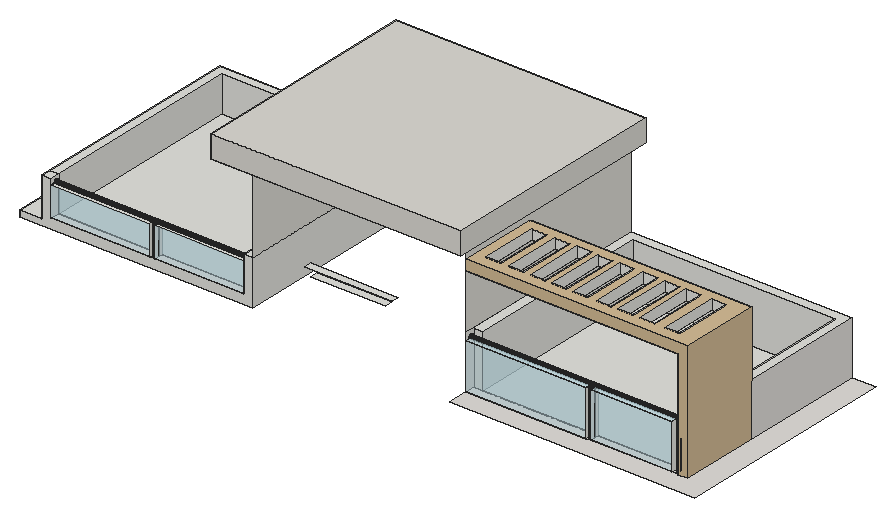
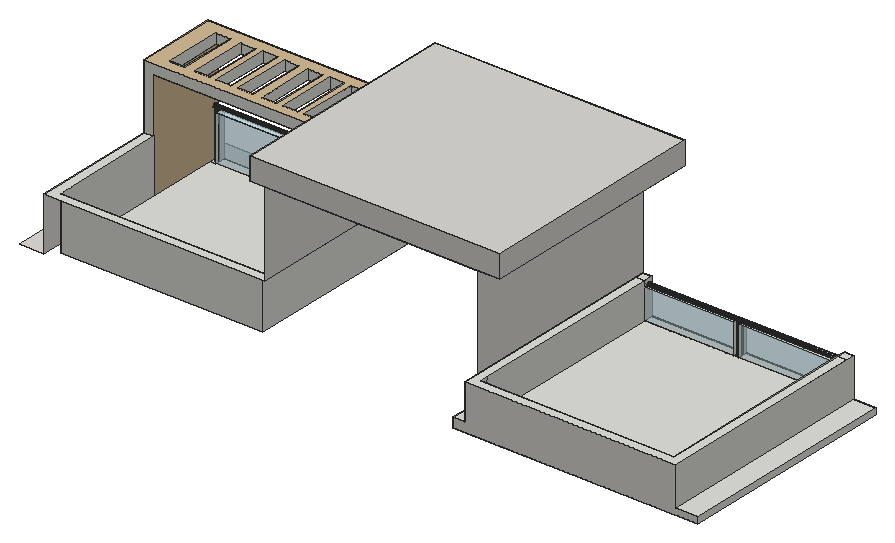
# SketchUp Ruby script. Lengths in inches.
U = 1.inch
M = Sketchup.active_model
def pt(a) = Geom::Point3d.new(a.map { |v| v * U })
def face(e, loops, mat)
  f = e.add_face(loops[0].map { |a| pt(a) })
  loops[1..].each { |l| e.add_face(l.map { |a| pt(a) }).erase! }
  f.material = f.back_material = mat if mat
  f
end
# faces: each face lists its corners as indices into pts; further lists are holes
def faces(e, pts, list, mat = nil) = list.each { |f| face(e, (f[0].is_a?(Array) ? f : [f]).map { |l| l.map { |i| pts[i] } }, mat) }
# xy, xz, yz: faces in a plane at the given z, y or x. An outline is a flat list of corners, or four numbers for a rectangle; further outlines are holes
def ring(l) = l.size == 4 ? [[l[0], l[1]], [l[2], l[1]], [l[2], l[3]], [l[0], l[3]]] : l.each_slice(2).to_a
def flat(e, list, mat, &to3) = list.each { |f| face(e, (f[0].is_a?(Array) ? f : [f]).map { |l| ring(l).map { |u, v| to3.(u, v) } }, mat) }
def xy(e, z, list, mat = nil) = flat(e, list, mat) { |x, y| [x, y, z] }
def xz(e, y, list, mat = nil) = flat(e, list, mat) { |x, z| [x, y, z] }
def yz(e, x, list, mat = nil) = flat(e, list, mat) { |y, z| [x, y, z] }
def lines(e, pts, list) = list.each { |a, b| e.add_line(pt(pts[a]), pt(pts[b])) }
# prism: a flat outline (further loops are holes) pulled along v
def prism(e, loops, v, mat = nil)
  f = face(e, loops, mat); d = Geom::Vector3d.new(v.map { |x| x * U })
  f.pushpull(f.normal.samedirection?(d) ? d.length : -d.length)
end
def box(e, o, s, mat = nil) = prism(e, [[o, [o[0] + s[0], o[1], o[2]], [o[0] + s[0], o[1] + s[1], o[2]], [o[0], o[1] + s[1], o[2]]]], [0, 0, s[2]], mat)
def at(x, y, z, deg = 0) = Geom::Transformation.translation(pt([x, y, z])) * Geom::Transformation.rotation(ORIGIN, Z_AXIS, deg.degrees)
def axes(o, x, y, z) = Geom::Transformation.new([*x, 0, *y, 0, *z, 0, *pt(o).to_a, 1])
def part(name) = M.definitions.add(name)
# library, detail: a bought-in or finely detailed component or shape, given as its bounding box
def library(name, o, s) = part(name).tap { |d| box(d.entities, o, s) }
def detail(e, o, s) = box(e.add_group.entities, o, s)
def put(e, d, t, mat = nil) = e.add_instance(d, t).tap { |i| i.material = mat if mat }
def group(e, t, mat = nil) = e.add_group.tap { |g| g.transformation = t; g.material = mat if mat }.entities
root = M.entities
M.materials.add("[Formica Beige]").color = [211, 187, 149]
M.materials.add("[Terrazzo Tile Accent]").color = [224, 221, 217]
M.materials.add("[Terrazzo Tile Light]").color = [219, 217, 210]
M.materials.add("[Translucent Glass Safety]").color = [204, 235, 244]
M.materials["[Translucent Glass Safety]"].alpha = 0.5
xy(root,573.6875,[[8.45,114.1,21.57,244.83],[21.57,114.1,21.57,244.83,152.39,244.83,152.39,235.11,145.58,235.11,145.58,114.1],[270.97,114.1,270.97,119.66,341.44,119.66,341.44,117.58,341.3125,117.27,341.27,116.91,341.3125,116.56,341.44,116.24,341.44,114.1],[341.44,114.1,344.2,114.1,344.2,119.66,341.44,119.66,341.44,117.58,341.45,117.6,341.67,117.88,341.95,118.1,342.29,118.24,342.64,118.29,343,118.24,343.33,118.1,343.61,117.88,343.83,117.6,343.97,117.27,344.02,116.91,343.97,116.56,343.83,116.22,343.61,115.9375,343.33,115.72,343,115.58,342.64,115.54,342.29,115.58,341.95,115.72,341.67,115.9375,341.45,116.22,341.44,116.24],[344.2,114.1,391.99,119.66],
  [[391.99,114.1,395.61,119.66],[393.42,116.1875,393.17,116.22,392.92,116.32,392.72,116.48,392.56,116.6875,392.46,116.93,392.42,117.1875,392.46,117.45,392.56,117.6875,392.72,117.89,392.92,118.05,393.17,118.15,393.42,118.1875,393.68,118.15,393.92,118.05,394.13,117.89,394.29,117.6875,394.39,117.45,394.42,117.1875,394.39,116.93,394.29,116.6875,394.13,116.48,393.92,116.32,393.68,116.22]],[342.64,115.54,342.29,115.58,341.95,115.72,341.67,115.9375,341.45,116.22,341.44,116.24,341.44,117.58,341.45,117.6,341.67,117.88,341.95,118.1,342.29,118.24,342.64,118.29,343,118.24,343.33,118.1,343.61,117.88,343.83,117.6,343.97,117.27,344.02,116.91,343.97,116.56,343.83,116.22,343.61,115.9375,343.33,115.72,343,115.58],[393.42,116.1875,393.17,116.22,392.92,116.32,392.72,116.48,392.56,116.6875,392.46,116.93,392.42,117.1875,392.46,117.45,392.56,117.6875,392.72,117.89,392.92,118.05,393.17,118.15,393.42,118.1875,393.68,118.15,393.92,118.05,394.13,117.89,394.29,117.6875,394.39,117.45,394.42,117.1875,394.39,116.93,394.29,116.6875,394.13,116.48,393.92,116.32,393.68,116.22],[341.44,116.24,341.3125,116.56,341.27,116.91,341.3125,117.27,341.44,117.58],[276.53,119.66,395.61,229.56]])
xy(root,573.6875,[[270.97,102.04,415.04,102.04,415.04,235.11,401.16,235.11,401.16,114.1,270.97,114.1]],"[Terrazzo Tile Accent]")
xy(root,577.14,[[8.45,114.1,21.57,244.83]])
xy(root,579.1875,[[26.86,114.1,84.93,119.4],[[84.93,114.1,87.68,119.4],[86.24,115.7,85.92,115.74,85.62,115.86,85.36,116.0625,85.16,116.32,85.04,116.625,84.99,116.95,85.04,117.27,85.16,117.57,85.36,117.83,85.62,118.03,85.92,118.15,86.24,118.2,86.57,118.15,86.87,118.03,87.13,117.83,87.33,117.57,87.45,117.27,87.49,116.95,87.45,116.625,87.33,116.32,87.13,116.0625,86.87,115.86,86.57,115.74]],[87.68,114.1,140.28,119.4],[86.24,115.7,85.92,115.74,85.62,115.86,85.36,116.0625,85.16,116.32,85.04,116.625,84.99,116.95,85.04,117.27,85.16,117.57,85.36,117.83,85.62,118.03,85.92,118.15,86.24,118.2,86.57,118.15,86.87,118.03,87.13,117.83,87.33,117.57,87.45,117.27,87.49,116.95,87.45,116.625,87.33,116.32,87.13,116.0625,86.87,115.86,86.57,115.74],[26.86,119.4,140.28,239.54]])
xy(root,579.1875,[[145.58,235.11,152.39,244.83]],"[Terrazzo Tile Accent]")
xy(root,596.84,[[26.86,114.1,84.93,116.21],[87.68,114.1,140.28,116.21],[26.86,116.21,84.93,117.71],[87.68,116.21,140.28,117.71],[26.86,117.71,84.93,119.4],
  [87.68,117.71,140.28,119.4]])
xy(root,597.4375,[[86.24,115.7,86.57,115.74,86.87,115.86,87.13,116.0625,87.33,116.32,87.45,116.625,87.49,116.95,87.45,117.27,87.33,117.57,87.13,117.83,86.87,118.03,86.57,118.15,86.24,118.2,85.92,118.15,85.62,118.03,85.36,117.83,85.16,117.57,85.04,117.27,84.99,116.95,85.04,116.625,85.16,116.32,85.36,116.0625,85.62,115.86,85.92,115.74]])
xy(root,600.1875,[[21.57,114.1,26.86,119.4],[140.28,114.1,145.58,119.4],[21.57,119.4,26.86,119.4,26.86,239.54,140.28,239.54,140.28,119.4,145.58,119.4,145.58,244.83,21.57,244.83]])
xy(root,600.1875,[[270.97,114.1,341.44,114.1,341.44,116.24,341.3125,116.56,341.27,116.91,341.3125,117.27,341.44,117.58,341.44,119.66,270.97,119.66],[344.2,114.1,391.99,119.66]],"[Translucent Glass Safety]")
xy(root,601.4375,[[393.42,116.1875,393.68,116.22,393.92,116.32,394.13,116.48,394.29,116.6875,394.39,116.93,394.42,117.1875,394.39,117.45,394.29,117.6875,394.13,117.89,393.92,118.05,393.68,118.15,393.42,118.1875,393.17,118.15,392.92,118.05,392.72,117.89,392.56,117.6875,392.46,117.45,392.42,117.1875,392.46,116.93,392.56,116.6875,392.72,116.48,392.92,116.32,393.17,116.22]])
xy(root,601.5625,[[342.64,115.54,343,115.58,343.33,115.72,343.61,115.9375,343.83,116.22,343.97,116.56,344.02,116.91,343.97,117.27,343.83,117.6,343.61,117.88,343.33,118.1,343,118.24,342.64,118.29,342.29,118.24,341.95,118.1,341.67,117.88,341.45,117.6,341.3125,117.27,341.27,116.91,341.3125,116.56,341.45,116.22,341.67,115.9375,341.95,115.72,342.29,115.58]])
xy(root,604.875,[[270.97,119.66,276.53,119.66,276.53,229.56,395.61,229.56,395.61,161.07,401.16,161.07,401.16,235.11,270.97,235.11]])
xy(root,605.45,[[183.08,109.54,227.11,114.1]])
xy(root,609.125,[[179.41,109.54,230.79,114.1]])
xy(root,637.49,[[[270.97,114.1,395.61,161.07],[315.57,120.98,324.26,155.17],[276.95,120.98,285.63,155.17],[290.32,120.98,299.01,155.17],[303.2,120.98,311.88,155.17],[342.01,120.98,350.7,155.17],[354.88,120.98,363.57,155.17],[367.45,120.98,376.13,155.17],[382.26,120.98,390.95,155.17],[328.2,120.98,336.88,155.17]]],"[Formica Beige]")
xy(root,643.4375,[[[270.97,114.1,401.16,161.07],[315.57,120.98,324.26,155.17],[276.95,120.98,285.63,155.17],[290.32,120.98,299.01,155.17],[303.2,120.98,311.88,155.17],[342.01,120.98,350.7,155.17],[354.88,120.98,363.57,155.17],[367.45,120.98,376.13,155.17],[382.26,120.98,390.95,155.17],[328.2,120.98,336.88,155.17]]],"[Formica Beige]")
xy(root,654.5625,[[145.58,114.1,270.97,235.11]])
xy(root,654.5625,[[133.02,99.04,133.02,235.11,145.58,235.11,145.58,114.1,270.97,114.1,270.97,235.11,279.72,235.11,279.72,99.04]],"[Formica Beige]")
xy(root,667.75,[[133.02,99.04,279.72,235.11]],"[Terrazzo Tile Light]")
xz(root,99.04,[[133.02,654.5625,279.72,667.75]],"[Terrazzo Tile Light]")
xz(root,114.1,[[8.45,573.6875,145.58,573.6875,145.58,600.1875,140.28,600.1875,140.28,579.1875,26.86,579.1875,26.86,600.1875,21.57,600.1875,21.57,577.14,8.45,577.14]])
xz(root,114.1,[[395.61,573.6875,401.16,573.6875,401.16,643.4375,270.97,643.4375,270.97,637.49,395.61,637.49]],"[Formica Beige]")
xz(root,114.1,[[270.97,573.6875,341.44,600.1875],[344.2,573.6875,391.99,600.1875],[26.86,579.1875,84.93,596.84],[87.68,579.1875,140.28,596.84]],"[Translucent Glass Safety]")
xz(root,119.4,[[26.86,579.1875,84.93,596.84],[87.68,579.1875,140.28,596.84]],"[Translucent Glass Safety]")
xz(root,119.66,[[270.97,573.6875,276.53,600.1875],[270.97,600.1875,276.53,604.875]])
xz(root,119.66,[[276.53,573.6875,341.44,600.1875],[344.2,573.6875,391.99,600.1875]],"[Translucent Glass Safety]")
xz(root,120.98,[[276.95,637.49,285.63,643.4375],[290.32,637.49,299.01,643.4375],[303.2,637.49,311.88,643.4375],[315.57,637.49,324.26,643.4375],[328.2,637.49,336.88,643.4375],
  [342.01,637.49,350.7,643.4375],[354.88,637.49,363.57,643.4375],[367.45,637.49,376.13,643.4375],[382.26,637.49,390.95,643.4375]])
xz(root,155.17,[[276.95,637.49,285.63,643.4375],[290.32,637.49,299.01,643.4375],[303.2,637.49,311.88,643.4375],[315.57,637.49,324.26,643.4375],[328.2,637.49,336.88,643.4375],
  [342.01,637.49,350.7,643.4375],[354.88,637.49,363.57,643.4375],[367.45,637.49,376.13,643.4375],[382.26,637.49,390.95,643.4375]])
xz(root,161.07,[[395.61,604.875,395.61,637.49,270.97,637.49,270.97,643.4375,401.16,643.4375,401.16,604.875]])
xz(root,229.56,[[276.53,573.6875,395.61,604.875]])
xz(root,235.11,[[145.58,573.6875,152.39,579.1875]])
xz(root,235.11,[[133.02,654.5625,279.72,667.75]],"[Terrazzo Tile Light]")
xz(root,239.54,[[26.86,579.1875,140.28,600.1875]])
xz(root,244.83,[[8.45,573.6875,8.45,577.14,21.57,577.14,21.57,600.1875,145.58,600.1875,145.58,579.1875,152.39,579.1875,152.39,573.6875]],"[Terrazzo Tile Accent]")
yz(root,8.45,[[114.1,573.6875,244.83,577.14]])
yz(root,21.57,[[114.1,577.14,244.83,600.1875]])
yz(root,26.86,[[114.1,579.1875,119.4,579.1875,119.4,596.84,117.71,596.84,117.49,596.67,117.23,596.57,116.96,596.53,116.68,596.57,116.43,596.67,116.21,596.84,114.1,596.84],[119.4,579.1875,239.54,600.1875],[116.96,596.53,116.68,596.57,116.43,596.67,116.21,596.84,117.71,596.84,117.49,596.67,117.23,596.57],[114.1,596.84,116.21,596.84,116.04,597.0625,115.93,597.32,115.9,597.59,115.93,597.87,116.04,598.125,116.21,598.35,116.43,598.51,116.68,598.62,116.96,598.66,117.23,598.62,117.49,598.51,117.71,598.35,117.88,598.125,117.99,597.87,118.02,597.59,117.99,597.32,117.88,597.0625,117.71,596.84,119.4,596.84,119.4,600.1875,114.1,600.1875]])
yz(root,84.93,[[114.1,579.1875,119.4,596.84]])
yz(root,87.68,[[114.1,579.1875,119.4,596.84]])
yz(root,133.02,[[99.04,654.5625,235.11,667.75]],"[Terrazzo Tile Light]")
yz(root,140.28,[[114.1,579.1875,119.4,579.1875,119.4,596.84,117.71,596.84,117.49,596.67,117.23,596.57,116.96,596.53,116.68,596.57,116.43,596.67,116.21,596.84,114.1,596.84],[119.4,579.1875,235.11,600.1875],[235.11,579.1875,239.54,600.1875],[116.96,596.53,117.23,596.57,117.49,596.67,117.71,596.84,116.21,596.84,116.43,596.67,116.68,596.57],[114.1,596.84,114.1,600.1875,119.4,600.1875,119.4,596.84,117.71,596.84,117.88,597.0625,117.99,597.32,118.02,597.59,117.99,597.87,117.88,598.125,117.71,598.35,117.49,598.51,117.23,598.62,116.96,598.66,116.68,598.62,116.43,598.51,116.21,598.35,116.04,598.125,115.93,597.87,115.9,597.59,115.93,597.32,116.04,597.0625,116.21,596.84],
  [116.21,596.84,117.71,596.84,117.88,597.0625,117.99,597.32,118.02,597.59,117.99,597.87,117.88,598.125,117.71,598.35,117.49,598.51,117.23,598.62,116.96,598.66,116.68,598.62,116.43,598.51,116.21,598.35,116.04,598.125,115.93,597.87,115.9,597.59,115.93,597.32,116.04,597.0625]])
yz(root,145.58,[[114.1,573.6875,235.11,600.1875]])
yz(root,145.58,[[235.11,579.1875,244.83,600.1875]],"[Terrazzo Tile Accent]")
yz(root,145.58,[[114.1,600.1875,235.11,654.5625]],"[Terrazzo Tile Light]")
yz(root,152.39,[[235.11,573.6875,244.83,579.1875]],"[Terrazzo Tile Accent]")
yz(root,270.97,[[114.1,573.6875,119.66,600.1875],[[114.1,600.1875,119.66,604.875],[116.79,600.81,116.52,600.84,116.26,600.95,116.04,601.12,115.87,601.34,115.76,601.59,115.73,601.87,115.76,602.14,115.87,602.4,116.04,602.62,116.26,602.79,116.52,602.89,116.79,602.93,117.07,602.89,117.32,602.79,117.54,602.62,117.71,602.4,117.82,602.14,117.85,601.87,117.82,601.59,117.71,601.34,117.54,601.12,117.32,600.95,117.07,600.84]],[116.79,600.81,116.52,600.84,116.26,600.95,116.04,601.12,115.87,601.34,115.76,601.59,115.73,601.87,115.76,602.14,115.87,602.4,116.04,602.62,116.26,602.79,116.52,602.89,116.79,602.93,117.07,602.89,117.32,602.79,117.54,602.62,117.71,602.4,117.82,602.14,117.85,601.87,117.82,601.59,117.71,601.34,117.54,601.12,117.32,600.95,117.07,600.84]])
yz(root,270.97,[[114.1,604.875,235.11,604.875,235.11,654.5625,114.1,654.5625,114.1,643.4375,161.07,643.4375,161.07,637.49,114.1,637.49]],"[Terrazzo Tile Light]")
yz(root,276.53,[[119.66,573.6875,229.56,604.875]])
yz(root,276.95,[[120.98,637.49,155.17,643.4375]])
yz(root,279.72,[[99.04,654.5625,235.11,667.75]],"[Terrazzo Tile Light]")
yz(root,285.63,[[120.98,637.49,155.17,643.4375]])
yz(root,290.32,[[120.98,637.49,155.17,643.4375]])
yz(root,299.01,[[120.98,637.49,155.17,643.4375]])
yz(root,303.2,[[120.98,637.49,155.17,643.4375]])
yz(root,311.88,[[120.98,637.49,155.17,643.4375]])
yz(root,315.57,[[120.98,637.49,155.17,643.4375]])
yz(root,324.26,[[120.98,637.49,155.17,643.4375]])
yz(root,328.2,[[120.98,637.49,155.17,643.4375]])
yz(root,336.88,[[120.98,637.49,155.17,643.4375]])
yz(root,341.44,[[114.1,573.6875,116.24,600.1875],[117.58,573.6875,119.66,600.1875]])
yz(root,342.01,[[120.98,637.49,155.17,643.4375]])
yz(root,344.2,[[114.1,573.6875,119.66,600.1875]])
yz(root,350.7,[[120.98,637.49,155.17,643.4375]])
yz(root,354.88,[[120.98,637.49,155.17,643.4375]])
yz(root,363.57,[[120.98,637.49,155.17,643.4375]])
yz(root,367.45,[[120.98,637.49,155.17,643.4375]])
yz(root,376.13,[[120.98,637.49,155.17,643.4375]])
yz(root,382.26,[[120.98,637.49,155.17,643.4375]])
yz(root,390.95,[[120.98,637.49,155.17,643.4375]])
yz(root,391.99,[[114.1,573.6875,119.66,600.1875]])
yz(root,395.61,[[161.07,573.6875,229.56,604.875]])
yz(root,395.61,[[[114.1,573.6875,161.07,637.49],[116.79,600.81,117.07,600.84,117.32,600.95,117.54,601.12,117.71,601.34,117.82,601.59,117.85,601.87,117.82,602.14,117.71,602.4,117.54,602.62,117.32,602.79,117.07,602.89,116.79,602.93,116.52,602.89,116.26,602.79,116.04,602.62,115.87,602.4,115.76,602.14,115.73,601.87,115.76,601.59,115.87,601.34,116.04,601.12,116.26,600.95,116.52,600.84]]],"[Formica Beige]")
yz(root,401.16,[[114.1,573.6875,161.07,643.4375]],"[Formica Beige]")
yz(root,401.16,[[161.07,573.6875,235.11,604.875]],"[Terrazzo Tile Accent]")
p = [[342.29,115.58,573.6875],[342.64,115.54,573.6875],[342.64,115.54,601.5625],[342.29,115.58,601.5625],[343,115.58,573.6875],[343,115.58,601.5625],
  [341.95,115.72,573.6875],[341.95,115.72,601.5625],[343.33,115.72,573.6875],[343.33,115.72,601.5625],[341.67,115.9375,573.6875],[341.67,115.9375,601.5625],
  [343.61,115.9375,573.6875],[343.61,115.9375,601.5625],[341.45,116.22,573.6875],[341.45,116.22,601.5625],[343.83,116.22,573.6875],[343.83,116.22,601.5625],
  [341.44,116.24,573.6875],[341.3125,116.56,601.5625],[341.3125,116.56,600.1875],[341.44,116.24,600.1875],[341.3125,116.56,573.6875],[343.97,116.56,573.6875],
  [343.97,116.56,601.5625],[392.92,116.32,573.6875],[393.17,116.22,573.6875],[393.17,116.22,601.4375],[392.92,116.32,601.4375],[393.42,116.1875,573.6875],
  [393.42,116.1875,601.4375],[393.68,116.22,573.6875],[393.68,116.22,601.4375],[393.92,116.32,573.6875],[393.92,116.32,601.4375],[392.72,116.48,573.6875],
  [392.72,116.48,601.4375],[394.13,116.48,573.6875],[394.13,116.48,601.4375],[392.56,116.6875,573.6875],[392.56,116.6875,601.4375],[394.29,116.6875,573.6875],
  [394.29,116.6875,601.4375],[341.27,116.91,573.6875],[341.27,116.91,600.1875],[344.02,116.91,573.6875],[344.02,116.91,601.5625],[392.46,116.93,573.6875],
  [392.46,116.93,601.4375],[394.39,116.93,573.6875],[394.39,116.93,601.4375],[341.3125,117.27,573.6875],[341.3125,117.27,600.1875],[343.97,117.27,573.6875],
  [343.97,117.27,601.5625],[392.42,117.1875,573.6875],[392.42,117.1875,601.4375],[394.42,117.1875,573.6875],[394.42,117.1875,601.4375],[392.46,117.45,573.6875],
  [392.46,117.45,601.4375],[394.39,117.45,573.6875],[394.39,117.45,601.4375],[341.45,117.6,573.6875],[341.44,117.58,573.6875],[341.44,117.58,600.1875],
  [341.3125,117.27,601.5625],[341.45,117.6,601.5625],[343.83,117.6,573.6875],[343.83,117.6,601.5625],[392.56,117.6875,573.6875],[392.56,117.6875,601.4375],
  [394.29,117.6875,573.6875],[394.29,117.6875,601.4375],[341.67,117.88,573.6875],[341.67,117.88,601.5625],[343.61,117.88,573.6875],[343.61,117.88,601.5625],
  [392.72,117.89,573.6875],[392.72,117.89,601.4375],[394.13,117.89,573.6875],[394.13,117.89,601.4375],[341.95,118.1,573.6875],[341.95,118.1,601.5625],
  [343.33,118.1,573.6875],[343.33,118.1,601.5625],[392.92,118.05,573.6875],[392.92,118.05,601.4375],[393.92,118.05,573.6875],[393.92,118.05,601.4375],
  [342.29,118.24,573.6875],[342.29,118.24,601.5625],[343,118.24,573.6875],[343,118.24,601.5625],[393.17,118.15,573.6875],[393.17,118.15,601.4375],
  [393.68,118.15,573.6875],[393.68,118.15,601.4375],[342.64,118.29,573.6875],[342.64,118.29,601.5625],[393.42,118.1875,573.6875],[393.42,118.1875,601.4375],
  [85.62,115.86,579.1875],[85.92,115.74,579.1875],[85.92,115.74,597.4375],[85.62,115.86,597.4375],[86.24,115.7,579.1875],[86.24,115.7,597.4375],
  [86.57,115.74,579.1875],[86.57,115.74,597.4375],[86.87,115.86,579.1875],[86.87,115.86,597.4375],[85.36,116.0625,579.1875],[85.36,116.0625,597.4375],
  [87.13,116.0625,579.1875],[87.13,116.0625,597.4375],[85.16,116.32,579.1875],[85.16,116.32,597.4375],[87.33,116.32,579.1875],[87.33,116.32,597.4375],
  [85.04,116.625,579.1875],[85.04,116.625,597.4375],[87.45,116.625,579.1875],[87.45,116.625,597.4375],[84.99,116.95,579.1875],[84.99,116.95,597.4375],
  [87.49,116.95,579.1875],[87.49,116.95,597.4375],[85.04,117.27,579.1875],[85.04,117.27,597.4375],[87.45,117.27,579.1875],[87.45,117.27,597.4375],
  [85.16,117.57,579.1875],[85.16,117.57,597.4375],[87.33,117.57,579.1875],[87.33,117.57,597.4375],[85.36,117.83,579.1875],[85.36,117.83,597.4375],
  [87.13,117.83,579.1875],[87.13,117.83,597.4375],[85.62,118.03,579.1875],[85.62,118.03,597.4375],[86.87,118.03,579.1875],[86.87,118.03,597.4375],
  [85.92,118.15,579.1875],[85.92,118.15,597.4375],[86.57,118.15,579.1875],[86.57,118.15,597.4375],[86.24,118.2,579.1875],[86.24,118.2,597.4375],
  [140.28,116.96,596.53],[140.28,116.68,596.57],[26.86,116.68,596.57],[26.86,116.96,596.53],[140.28,117.23,596.57],[26.86,117.23,596.57],
  [140.28,116.43,596.67],[26.86,116.43,596.67],[140.28,117.49,596.67],[26.86,117.49,596.67],[140.28,116.21,596.84],[87.68,116.21,596.84],
  [84.93,116.21,596.84],[26.86,116.21,596.84],[140.28,117.71,596.84],[26.86,117.71,596.84],[84.93,117.71,596.84],[87.68,117.71,596.84],
  [140.28,116.04,597.0625],[26.86,116.04,597.0625],[140.28,117.88,597.0625],[26.86,117.88,597.0625],[140.28,115.93,597.32],[26.86,115.93,597.32],
  [140.28,117.99,597.32],[26.86,117.99,597.32],[140.28,115.9,597.59],[26.86,115.9,597.59],[140.28,118.02,597.59],[26.86,118.02,597.59],
  [140.28,115.93,597.87],[26.86,115.93,597.87],[140.28,117.99,597.87],[26.86,117.99,597.87],[140.28,116.04,598.125],[26.86,116.04,598.125],
  [140.28,117.88,598.125],[26.86,117.88,598.125],[140.28,116.21,598.35],[26.86,116.21,598.35],[140.28,117.71,598.35],[26.86,117.71,598.35],
  [140.28,116.43,598.51],[26.86,116.43,598.51],[140.28,117.49,598.51],[26.86,117.49,598.51],[140.28,116.68,598.62],[26.86,116.68,598.62],
  [140.28,117.23,598.62],[26.86,117.23,598.62],[140.28,116.96,598.66],[26.86,116.96,598.66],[341.27,116.91,601.5625],[270.97,116.26,600.95],
  [270.97,116.52,600.84],[395.61,116.52,600.84],[395.61,116.26,600.95],[270.97,116.79,600.81],[395.61,116.79,600.81],[270.97,117.07,600.84],
  [395.61,117.07,600.84],[270.97,117.32,600.95],[395.61,117.32,600.95],[270.97,116.04,601.12],[395.61,116.04,601.12],[270.97,117.54,601.12],
  [395.61,117.54,601.12],[270.97,115.87,601.34],[395.61,115.87,601.34],[270.97,117.71,601.34],[395.61,117.71,601.34],[270.97,115.76,601.59],
  [395.61,115.76,601.59],[270.97,117.82,601.59],[395.61,117.82,601.59],[270.97,115.73,601.87],[395.61,115.73,601.87],[270.97,117.85,601.87],
  [395.61,117.85,601.87],[270.97,115.76,602.14],[395.61,115.76,602.14],[270.97,117.82,602.14],[395.61,117.82,602.14],[270.97,115.87,602.4],
  [395.61,115.87,602.4],[270.97,117.71,602.4],[395.61,117.71,602.4],[270.97,116.04,602.62],[395.61,116.04,602.62],[270.97,117.54,602.62],
  [395.61,117.54,602.62],[270.97,116.26,602.79],[395.61,116.26,602.79],[270.97,117.32,602.79],[395.61,117.32,602.79],[270.97,116.52,602.89],
  [395.61,116.52,602.89],[270.97,117.07,602.89],[395.61,117.07,602.89],[270.97,116.79,602.93],[395.61,116.79,602.93]]
faces(root,p,[[0,1,2,3],[1,4,5,2],[6,0,3,7],[4,8,9,5],[10,6,7,11],[8,12,13,9],[14,10,11,15],[12,16,17,13],
  [18,14,15,19,20,21],[22,18,21,20],[16,23,24,17],[25,26,27,28],[26,29,30,27],[29,31,32,30],[31,33,34,32],[35,25,28,36],
  [33,37,38,34],[39,35,36,40],[37,41,42,38],[43,22,20,44],[23,45,46,24],[47,39,40,48],[41,49,50,42],[51,43,44,52],
  [45,53,54,46],[55,47,48,56],[49,57,58,50],[59,55,56,60],[57,61,62,58],[63,64,65,52,66,67],[64,51,52,65],[53,68,69,54],
  [70,59,60,71],[61,72,73,62],[74,63,67,75],[68,76,77,69],[78,70,71,79],[72,80,81,73],[82,74,75,83],[76,84,85,77],
  [86,78,79,87],[80,88,89,81],[90,82,83,91],[84,92,93,85],[94,86,87,95],[88,96,97,89],[98,90,91,99],[92,98,99,93],
  [100,94,95,101],[96,100,101,97],[102,103,104,105],[103,106,107,104],[106,108,109,107],[108,110,111,109],[112,102,105,113],[110,114,115,111],
  [116,112,113,117],[114,118,119,115],[120,116,117,121],[118,122,123,119],[124,120,121,125],[122,126,127,123],[128,124,125,129],[126,130,131,127],
  [132,128,129,133],[130,134,135,131],[136,132,133,137],[134,138,139,135],[140,136,137,141],[138,142,143,139],[144,140,141,145],[142,146,147,143],
  [148,144,145,149],[146,148,149,147],[150,151,152,153],[154,150,153,155],[151,156,157,152],[158,154,155,159],[156,160,161,162,163,157],[164,158,159,165,166,167],
  [160,168,169,163,162,161],[170,164,167,166,165,171],[168,172,173,169],[174,170,171,175],[172,176,177,173],[178,174,175,179],[176,180,181,177],[182,178,179,183],
  [180,184,185,181],[186,182,183,187],[184,188,189,185],[190,186,187,191],[188,192,193,189],[194,190,191,195],[192,196,197,193],[198,194,195,199],
  [196,200,201,197],[200,198,199,201],[202,44,20,19],[66,52,44,202],[203,204,205,206],[204,207,208,205],[207,209,210,208],[209,211,212,210],
  [213,203,206,214],[211,215,216,212],[217,213,214,218],[215,219,220,216],[221,217,218,222],[219,223,224,220],[225,221,222,226],[223,227,228,224],
  [229,225,226,230],[227,231,232,228],[233,229,230,234],[231,235,236,232],[237,233,234,238],[235,239,240,236],[241,237,238,242],[239,243,244,240],
  [245,241,242,246],[243,247,248,244],[249,245,246,250],[247,249,250,248]])
